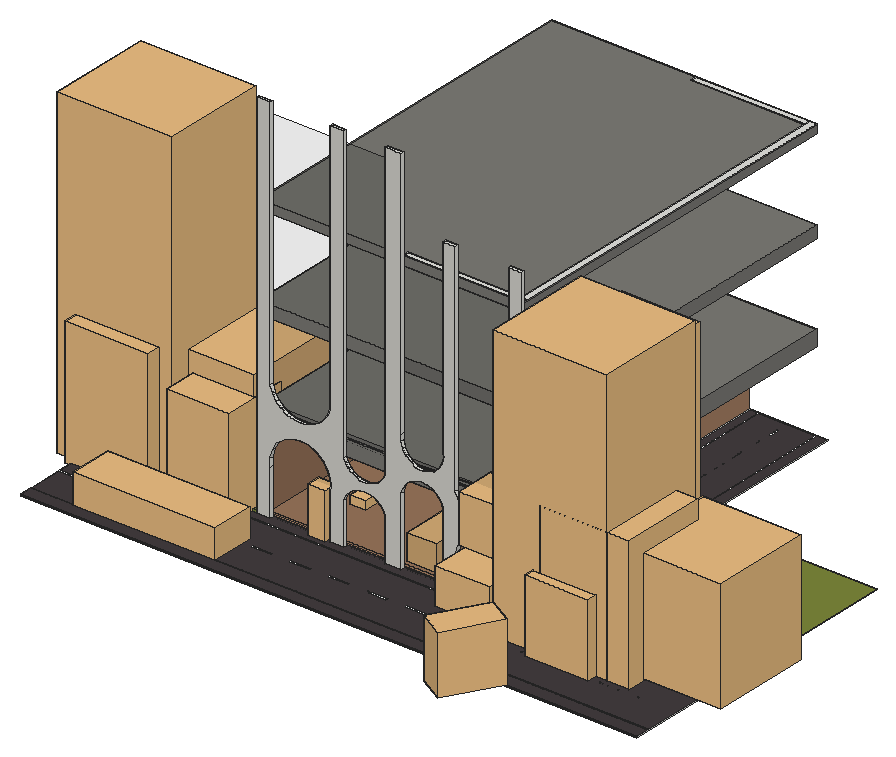
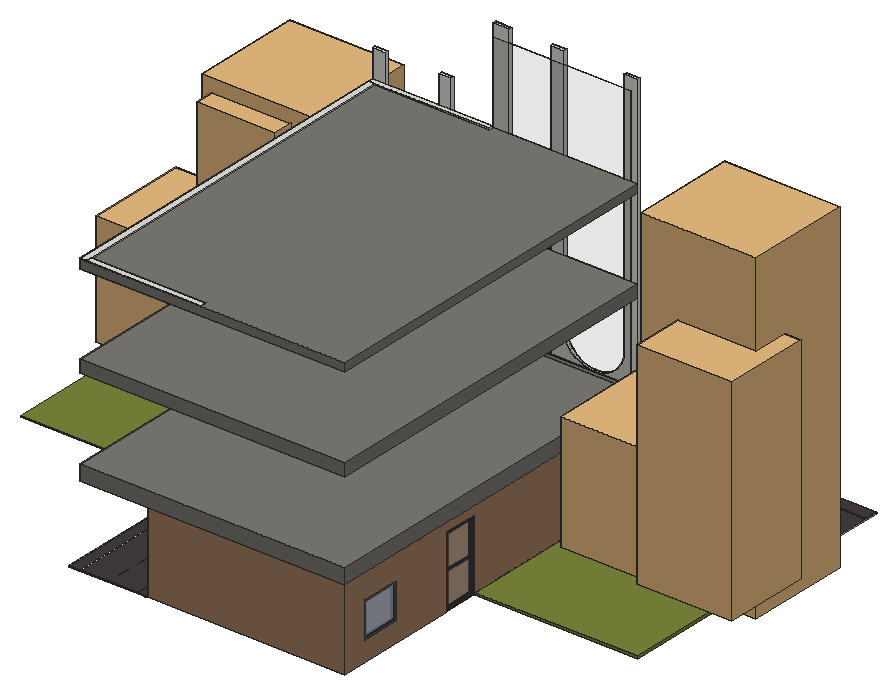
# SketchUp Ruby script. Lengths in inches.
U = 1.inch
M = Sketchup.active_model
def pt(a) = Geom::Point3d.new(a.map { |v| v * U })
def face(e, loops, mat)
  f = e.add_face(loops[0].map { |a| pt(a) })
  loops[1..].each { |l| e.add_face(l.map { |a| pt(a) }).erase! }
  f.material = f.back_material = mat if mat
  f
end
# faces: each face lists its corners as indices into pts; further lists are holes
def faces(e, pts, list, mat = nil) = list.each { |f| face(e, (f[0].is_a?(Array) ? f : [f]).map { |l| l.map { |i| pts[i] } }, mat) }
# xy, xz, yz: faces in a plane at the given z, y or x. An outline is a flat list of corners, or four numbers for a rectangle; further outlines are holes
def ring(l) = l.size == 4 ? [[l[0], l[1]], [l[2], l[1]], [l[2], l[3]], [l[0], l[3]]] : l.each_slice(2).to_a
def flat(e, list, mat, &to3) = list.each { |f| face(e, (f[0].is_a?(Array) ? f : [f]).map { |l| ring(l).map { |u, v| to3.(u, v) } }, mat) }
def xy(e, z, list, mat = nil) = flat(e, list, mat) { |x, y| [x, y, z] }
def xz(e, y, list, mat = nil) = flat(e, list, mat) { |x, z| [x, y, z] }
def yz(e, x, list, mat = nil) = flat(e, list, mat) { |y, z| [x, y, z] }
def lines(e, pts, list) = list.each { |a, b| e.add_line(pt(pts[a]), pt(pts[b])) }
# prism: a flat outline (further loops are holes) pulled along v
def prism(e, loops, v, mat = nil)
  f = face(e, loops, mat); d = Geom::Vector3d.new(v.map { |x| x * U })
  f.pushpull(f.normal.samedirection?(d) ? d.length : -d.length)
end
def box(e, o, s, mat = nil) = prism(e, [[o, [o[0] + s[0], o[1], o[2]], [o[0] + s[0], o[1] + s[1], o[2]], [o[0], o[1] + s[1], o[2]]]], [0, 0, s[2]], mat)
def at(x, y, z, deg = 0) = Geom::Transformation.translation(pt([x, y, z])) * Geom::Transformation.rotation(ORIGIN, Z_AXIS, deg.degrees)
def axes(o, x, y, z) = Geom::Transformation.new([*x, 0, *y, 0, *z, 0, *pt(o).to_a, 1])
def part(name) = M.definitions.add(name)
# library, detail: a bought-in or finely detailed component or shape, given as its bounding box
def library(name, o, s) = part(name).tap { |d| box(d.entities, o, s) }
def detail(e, o, s) = box(e.add_group.entities, o, s)
def put(e, d, t, mat = nil) = e.add_instance(d, t).tap { |i| i.material = mat if mat }
def group(e, t, mat = nil) = e.add_group.tap { |g| g.transformation = t; g.material = mat if mat }.entities
root = M.entities
M.materials.add("Bricks A04 100cm").color = [167, 128, 100]
M.materials.add("Concrete Grey 06 100cm").color = [123, 122, 117]
M.materials.add("Concrete Rough Rocks 16-07 100cm\#1").color = [212, 211, 204]
M.materials.add("Glass Clear 001").color = [0, 0, 0]
M.materials["Glass Clear 001"].alpha = 0.1
M.materials.add("Grass E 200cm\#1").color = [123, 134, 58]
M.materials.add("Windows").color = [58, 58, 58]
M.materials.add("[Asphalt_New]").color = [67, 60, 62]
M.materials.add("[Color_000]").color = [255, 255, 255]
M.materials.add("[Color_006]").color = [86, 86, 86]
M.materials.add("[Translucent Glass Gray]1").color = [128, 128, 128]
M.materials["[Translucent Glass Gray]1"].alpha = 0.5
M.materials.add("[Translucent_Glass_Gray]1").color = [167, 187, 214]
M.materials["[Translucent_Glass_Gray]1"].alpha = 0.8
c1 = library("Schefflera arboricola 004",[-66.29,-60.4,-0.79],[131.92,126.97,148.56])
c2 = library("Schefflera arboricola 003",[-47.85,-46.83,-0.79],[92.88,94.95,107.86])
c3 = part("Window+06")
g1 = group(c3.entities,at(-11,5.5,0,-90))
xy(g1,0,[[0,11,5.5,35]],"Windows")
xy(g1,2,[[0,13,5.5,33]],"Windows")
xy(g1,53,[[0,13,5.5,33]],"Windows")
xy(g1,55,[[0,11,5.5,35]],"Windows")
xz(g1,11,[[0,0,5.5,55]],"Windows")
xz(g1,13,[[0,2,5.5,53]],"Windows")
xz(g1,33,[[0,2,5.5,53]],"Windows")
xz(g1,35,[[0,0,5.5,55]],"Windows")
yz(g1,0,[[[11,0,35,55],[13,2,33,53]]],"Windows")
yz(g1,5.5,[[[11,0,35,55],[13,2,33,53]]],"Windows")
g2 = group(g1,at(2.75,2,2))
xy(g2,0,[[0,11,2,31]],"Windows")
xy(g2,1,[[0,12,1,30],[1,12,2,30]],"Windows")
xy(g2,25,[[0,12,1,30],[1,12,2,30]],"Windows")
xy(g2,26,[[0,11,2,31]],"Windows")
xz(g2,11,[[0,0,2,26]],"Windows")
xz(g2,12,[[0,1,1,25],[1,1,2,25]],"Windows")
xz(g2,30,[[0,1,1,25],[1,1,2,25]],"Windows")
xz(g2,31,[[0,0,2,26]],"Windows")
yz(g2,0,[[[11,0,31,26],[12,1,30,25]]],"Windows")
yz(g2,1,[[12,1,30,25]],"[Translucent Glass Gray]1")
yz(g2,2,[[[11,0,31,26],[12,1,30,25]]],"Windows")
g3 = group(g1,at(0.75,2,27))
xy(g3,0,[[0,11,2,31]],"Windows")
xy(g3,1,[[0,12,1,30],[1,12,2,30]],"Windows")
xy(g3,25,[[0,12,1,30],[1,12,2,30]],"Windows")
xy(g3,26,[[0,11,2,31]],"Windows")
xz(g3,11,[[0,0,2,26]],"Windows")
xz(g3,12,[[0,1,1,25],[1,1,2,25]],"Windows")
xz(g3,30,[[0,1,1,25],[1,1,2,25]],"Windows")
xz(g3,31,[[0,0,2,26]],"Windows")
yz(g3,0,[[[11,0,31,26],[12,1,30,25]]],"Windows")
yz(g3,1,[[12,1,30,25]],"[Translucent Glass Gray]1")
yz(g3,2,[[[11,0,31,26],[12,1,30,25]]],"Windows")
c4 = library("Hugh 001 Standing",[-12.24,-10.14,0],[24.44,20.33,67.86])
c5 = library("Jalen Walking 001",[-18.74,-36.02,0],[37.48,72.04,73.58])
c6 = library("Car 034",[-40.54,-85.05,-1.09],[81.08,168.69,53.52])
c7 = part("Untitled (6)")
xy(c7.entities,0,[[-437.53,-1998.08,-389.53,356.87],[[-383.53,-1998.08,-383.53,356.87,-256.03,356.87,-256.03,283.28,-250.03,283.28,-250.03,356.87,-124.03,356.87,-124.03,-1998.08],[-256.03,136.09,-250.03,209.6875],[-256.03,-158.28,-250.03,-84.68],[-256.03,-599.83,-250.03,-526.24],[-256.03,-11.09,-250.03,62.5],[-256.03,-452.64,-250.03,-379.05],[-256.03,-747.01,-250.03,-673.42],[-256.03,-305.46,-250.03,-231.87],[-256.03,-1630.12,-250.03,-1556.53],[-256.03,-1482.93,-250.03,-1409.34],[-256.03,-1335.75,-250.03,-1262.16],[-256.03,-894.2,-250.03,-820.6],[-256.03,-1924.49,-250.03,-1850.89],[-256.03,-1188.57,-250.03,-1114.97],[-256.03,-1777.3,-250.03,-1703.71],[-256.03,-1041.38,-250.03,-967.79]],[-118.03,-1998.08,-70.03,356.87]],"[Asphalt_New]")
xy(c7.entities,0,[[-389.53,-1998.08,-383.53,356.87],[-124.03,-1998.08,-118.03,356.87],[-256.03,-1924.49,-250.03,-1850.89],[-256.03,-1777.3,-250.03,-1703.71],[-256.03,-1630.12,-250.03,-1556.53],
  [-256.03,-1482.93,-250.03,-1409.34],[-256.03,-1335.75,-250.03,-1262.16],[-256.03,-1188.57,-250.03,-1114.97],[-256.03,-1041.38,-250.03,-967.79],[-256.03,-894.2,-250.03,-820.6],
  [-256.03,-747.01,-250.03,-673.42],[-256.03,-599.83,-250.03,-526.24],[-256.03,-452.64,-250.03,-379.05],[-256.03,-305.46,-250.03,-231.87],[-256.03,-158.28,-250.03,-84.68],
  [-256.03,-11.09,-250.03,62.5],[-256.03,136.09,-250.03,209.6875],[-256.03,283.28,-250.03,356.87]],"[Color_000]")
c8 = library("Reception desk",[23.57,0,0],[37.45,80.71,54.72])
c9 = part("BIC_Bike Shop - Window - Small")
xy(c9.entities,-8,[[[0,0,36,36],[2,2,34,34]]],"[Color_006]")
xy(c9.entities,-4,[[2,2,34,34]],"[Translucent_Glass_Gray]1")
xy(c9.entities,0,[[[0,0,36,36],[2,2,34,34]]],"[Color_006]")
xz(c9.entities,0,[[0,-8,36,0]],"[Color_006]")
xz(c9.entities,2,[[2,-8,34,-4],[2,-4,34,0]],"[Color_006]")
xz(c9.entities,34,[[2,-8,34,-4],[2,-4,34,0]],"[Color_006]")
xz(c9.entities,36,[[0,-8,36,0]],"[Color_006]")
yz(c9.entities,0,[[0,-8,36,0]],"[Color_006]")
yz(c9.entities,2,[[2,-8,34,-4],[2,-4,34,0]],"[Color_006]")
yz(c9.entities,34,[[2,-8,34,-4],[2,-4,34,0]],"[Color_006]")
yz(c9.entities,36,[[0,-8,36,0]],"[Color_006]")
c10 = library("Dome Light",[-12,-12,0],[24,24,12])
c11 = library("Untitled+(35)",[-36.2,-34.81,25.37],[51.5,58.42,71.3])
box(root,[0.025,0,0],[911.788,140.625,1.3125])
box(root,[0,136.481,1.369],[240.0625,305,3.687],"Grass E 200cm\#1")
xy(root,1.369,[[533.3125,141.106,648.125,681.606],[648.125,141.106,648.4375,441.575]])
xy(root,1.369,[[648.4375,141.106,911.8125,441.575]],"Grass E 200cm\#1")
xy(root,2.306,[[533.3125,141.106,648.125,681.606]])
xy(root,3.056,[[648.4375,141.106,911.8125,441.575]],"Grass E 200cm\#1")
xy(root,140.053,[[247.445,141.106,612.5,150.106]],"Glass Clear 001")
xy(root,144.302,[[249.0625,141.606,453.445,141.606,612.5,150.106,247.445,150.106]],"Glass Clear 001")
xy(root,414.5625,[[631.5625,141.106,622.077,148.731,631.5625,148.731]])
xy(root,416.25,[[453.5,141.106,631.5625,141.106,631.5625,148.732,622.077,148.732,453.5,148.731]])
xy(root,534.5625,[[249.0625,141.106,453.445,141.606]],"Glass Clear 001")
xz(root,140.883,[[453.5,141.727,612.5,401.8125]],"Glass Clear 001")
xz(root,141.106,[[533.3125,1.369,648.125,2.306]])
xz(root,141.106,[[631.5625,414.5625,631.5625,416.25,453.5,416.25]],"Concrete Grey 06 100cm")
xz(root,141.106,[[247.445,140.053,249.0625,140.053,247.445,144.302]],"Glass Clear 001")
xz(root,141.606,[[249.0625,144.302,453.445,534.5625]],"Glass Clear 001")
xz(root,144.219,[[248.63,1.8125,513.626,119.9375]],"Glass Clear 001")
xz(root,148.731,[[622.077,414.5625,631.5625,414.929]])
xz(root,148.732,[[622.077,415.0625,631.5625,416.25]])
xz(root,150.106,[[247.445,140.053,612.5,144.302]],"Glass Clear 001")
xz(root,441.575,[[648.4375,1.369,911.8125,3.056]],"Grass E 200cm\#1")
xz(root,681.606,[[533.3125,1.369,648.125,2.306]])
yz(root,247.445,[[141.106,140.053,150.106,144.302]],"Glass Clear 001")
yz(root,249.0625,[[141.106,140.053,141.106,534.5625,141.606,534.5625,141.606,144.302]],"Glass Clear 001")
yz(root,453.445,[[141.106,140.053,141.606,144.302,141.606,534.5625,141.106,534.5625]],"Glass Clear 001")
yz(root,453.5,[[140.883,401.8125,141.106,416.25,148.731,416.25,148.731,414.5625]])
yz(root,533.3125,[[141.106,1.369,681.606,2.306]])
yz(root,612.5,[[141.106,140.053,150.106,140.053,150.106,144.302,140.883,141.727]],"Glass Clear 001")
yz(root,622.077,[[681.105,413.821,148.731,414.5625,148.731,414.929,148.732,415.0625,148.733,416.25,672.071,415.521,680.233,415.51,681.107,415.509,681.106,414.635]])
yz(root,631.5625,[[681.105,413.821,681.107,415.509,148.733,416.25,148.732,415.0625,148.731,414.929,148.731,414.5625],[141.106,414.5625,148.731,414.5625,148.731,414.929,148.732,415.0625,148.732,416.25,141.106,416.25]],"Concrete Grey 06 100cm")
yz(root,648.125,[[141.106,1.369,681.606,2.306]])
yz(root,648.4375,[[141.106,1.369,441.575,3.056]],"Grass E 200cm\#1")
p = [[453.445,141.106,140.053],[453.5,140.883,141.727],[453.445,141.606,144.302],[453.5,141.106,140.053],[612.5,141.106,140.053],[612.5,140.883,141.727],
  [247.445,141.106,144.302],[249.0625,141.106,140.053],[247.445,150.106,144.302],[249.0625,141.606,144.302],[612.5,150.106,144.302],[453.5,140.883,401.8125],
  [453.5,148.731,414.5625],[622.077,148.731,414.5625],[612.5,140.883,401.8125],[622.082,672.069,414.648],[453.817,672.068,413.701],[453.817,681.105,413.689],
  [622.077,681.106,414.635],[622.082,681.106,414.635],[622.082,680.232,414.636],[622.077,672.071,415.521],[453.8125,672.069,414.575],[453.8125,681.106,414.5625],
  [622.077,681.107,415.509],[622.077,681.105,413.821],[631.5625,681.105,413.821],[631.5625,148.731,414.5625],[631.5625,681.107,415.509],[622.077,148.731,414.929],
  [631.5625,148.731,414.929],[453.5,148.731,416.25],[622.077,148.732,416.25],[622.077,148.732,415.0625],[622.077,680.233,415.51],[631.5625,148.732,415.0625],
  [631.5625,148.733,416.25],[622.077,148.733,416.25],[0,-122.738,5.056],[0,-122.738,1.744]]
faces(root,p,[[0,1,2],[1,0,3],[3,4,5,1],[6,7,8],[9,8,7],[0,2,9,7],[1,10,2],[5,10,1]],"Glass Clear 001")
faces(root,p,[[11,12,13,14],[15,16,17,18,19,20],[21,22,16,15],[22,23,17,16],[23,24,18,17],[13,25,26,27],[25,18,19,24,28,26],[29,30,27,13,12,31,32,33],
  [22,21,34,24,23],[34,21,15,20],[24,34,20,19],[18,24,19],[29,30,35,33],[33,35,36,37],[34,21,37,36,28,24]])
lines(root,p,[[38,39]])
put(root,c1,axes([688.01,171.53,-13.56],[0.7936,0,0],[0,0.7936,0],[0,0,1.69965]))
put(root,c1,axes([47.65,188.84,-5.3],[1.2932,0,0],[0,1.22,0],[0,0,3.2208]))
put(root,c1,axes([769.6,141.11,0.27],[1,0,0],[0,1,0],[0,0,1.34]))
put(root,c1,axes([151.57,215.65,0.16],[1.2,0,0],[0,1.2,0],[0,0,1.2]))
put(root,c2,axes([53.78,141.01,0.58],[1.32,0,0],[0,1,0],[0,0,1.73203]))
put(root,c2,axes([188.3,141.01,0.31],[1,0,0],[0,1,0],[0,0,1.39]))
put(root,c1,axes([718.9,158.02,1.8125],[1.28,0,0],[0,1.28,0],[0,0,2.74138]))
put(root,c2,at(740.74,113.62,2))
put(root,c3,axes([242.3125,494.89,1.37],[0,-2.22917,0],[0.375,0,0],[0,0,1.92841]))
g4 = group(root,at(138.3125,141.11,0))
xy(g4,1.37,[[377.5625,-0.5,377.5625,531,110.75,531,110.75,353.78,101.75,353.78,101.75,540,393.52,540,393.52,-0.5],[101.75,0,110.75,300.47],[110.75,0,377.5625,9],[110.75,9,377.5625,531]],"Bricks A04 100cm")
xy(g4,30.4375,[[101.75,444.5,110.75,505.8125]],"Bricks A04 100cm")
xy(g4,85.12,[[101.75,444.5,110.75,505.8125]],"Bricks A04 100cm")
xy(g4,108.18,[[101.75,300.47,110.75,353.78]],"Bricks A04 100cm")
xy(g4,119.99,[[377.5625,-0.5,393.52,-0.5,393.52,540,101.75,540,101.75,0,110.75,0,110.75,531,377.5625,531]],"Bricks A04 100cm")
xz(g4,-0.5,[[377.5625,1.37,393.52,119.99]],"Bricks A04 100cm")
xz(g4,0,[[101.75,1.37,110.75,119.99]],"Bricks A04 100cm")
xz(g4,300.47,[[101.75,1.37,110.75,108.18]],"Bricks A04 100cm")
xz(g4,353.78,[[101.75,1.37,110.75,108.18]],"Bricks A04 100cm")
xz(g4,444.5,[[101.75,30.4375,110.75,85.12]],"Bricks A04 100cm")
xz(g4,505.8125,[[101.75,30.4375,110.75,85.12]],"Bricks A04 100cm")
xz(g4,531,[[110.75,1.37,377.5625,119.99]],"Bricks A04 100cm")
xz(g4,540,[[101.75,1.37,393.52,119.99]],"Bricks A04 100cm")
yz(g4,101.75,[[[0,1.37,0,119.99,540,119.99,540,1.37,353.78,1.37,353.78,108.18,300.47,108.18,300.47,1.37],[444.5,30.4375,505.8125,85.12]]],"Bricks A04 100cm")
yz(g4,110.75,[[0,1.37,9,119.99],[[9,1.37,300.47,1.37,300.47,108.18,353.78,108.18,353.78,1.37,531,1.37,531,119.99,9,119.99],[444.5,30.4375,505.8125,85.12]]],"Bricks A04 100cm")
yz(g4,377.5625,[[-0.5,1.37,531,119.99]],"Bricks A04 100cm")
yz(g4,393.52,[[-0.5,1.37,540,119.99]],"Bricks A04 100cm")
g5 = group(root,at(1099.8125,-728.61,1.37))
xy(g5,0,[[-859.75,865.09,-839.625,869.72],[-750.875,865.09,-731,869.72],[-669.5625,865.09,-646,869.72],[-584.125,865.09,-566.5,869.72]])
xy(g5,455.76,[[-584.125,865.09,-566.1875,869.72],[-487.75,865.09,-468,869.72]])
xy(g5,550.82,[[-859.75,865.09,-839.625,869.72],[-750.875,865.09,-731,869.72],[-669.5625,865.09,-646,869.72]])
xz(g5,865.09,[[-859.75,0,-839.625,0,-839.625,66.75,-839.78,79.63,-836.27,92.02,-829.38,102.91,-819.69,111.4,-808,116.78,-795.25,118.63,-782.5,116.78,-770.8,111.4,-761.11,102.91,-754.23,92.02,-750.72,79.63,-750.875,66.75,-750.875,0,-731,0,-731,62.4375,-728.15,68.47,-724.125,73.8,-719.1,78.2,-713.28,81.48,-706.92,83.5,-700.28,84.1875,-693.64,83.5,-687.28,81.48,-681.46,78.2,-676.4375,73.8,-672.41,68.47,-669.5625,62.4375,-669.5625,0,-646,0,-646,101.625,-643.7,108.39,-639.95,114.47,-634.93,119.55,-628.9,123.38,-622.16,125.76,-615.0625,126.5625,-607.96,125.76,-601.23,123.38,-595.19,119.55,-590.17,114.47,-586.42,108.39,-584.125,101.625,-584.125,0,-566.5,0,-566.5,38.9375,-565.37,50.2,-562.02,61.02,-556.6,70.95,-549.31,79.61,-540.44,86.65,-530.36,91.79,-519.45,94.82,-508.16,95.625,-496.94,94.17,-486.22,90.52,-476.45,84.8125,-468,77.28,-468,455.76,-487.75,455.76,-487.75,132.21,-491.16,124.22,-496.1875,117.13,-502.59,111.26,-510.08,106.87,-518.33,104.15,-526.97,103.23,-535.61,104.15,-543.86,106.87,-551.35,111.26,-557.75,117.13,-562.77,124.22,-566.1875,132.21,-566.1875,455.76,-584.125,455.76,-584.125,179.13,-583.7,169.91,-585.97,160.96,-590.73,153.05,-597.58,146.86,-605.93,142.92,-615.0625,141.57,-624.19,142.92,-632.54,146.86,-639.39,153.05,-644.16,160.96,-646.42,169.91,-646,179.13,-646,550.82,-669.5625,550.82,-669.5625,118.63,-672.23,112.36,-676.15,106.8,-681.17,102.1875,-687.04,98.74,-693.51,96.6,-700.28,95.88,-707.05,96.6,-713.52,98.74,-719.39,102.1875,-724.41,106.8,-728.33,112.36,-731,118.63,-731,550.82,-750.875,550.82,-750.875,176.63,-754.3,167.08,-759.76,158.53,-766.97,151.39,-775.58,146.03,-785.17,142.7,-795.25,141.57,-805.33,142.7,-814.92,146.03,-823.53,151.39,-830.74,158.53,-836.19,167.08,-839.625,176.63,-839.625,550.82,-859.75,550.82]],"Concrete Rough Rocks 16-07 100cm\#1")
xz(g5,869.72,[[-859.75,0,-859.75,550.82,-839.625,550.82,-839.625,176.63,-836.19,167.08,-830.74,158.53,-823.53,151.39,-814.92,146.03,-805.33,142.7,-795.25,141.57,-785.17,142.7,-775.58,146.03,-766.97,151.39,-759.76,158.53,-754.3,167.08,-750.875,176.63,-750.875,550.82,-731,550.82,-731,118.63,-728.33,112.36,-724.41,106.8,-719.39,102.1875,-713.52,98.74,-707.05,96.6,-700.28,95.88,-693.51,96.6,-687.04,98.74,-681.17,102.1875,-676.15,106.8,-672.23,112.36,-669.5625,118.63,-669.5625,550.82,-646,550.82,-646,179.13,-646.42,169.91,-644.16,160.96,-639.39,153.05,-632.54,146.86,-624.19,142.92,-615.0625,141.57,-605.93,142.92,-597.58,146.86,-590.73,153.05,-585.97,160.96,-583.7,169.91,-584.125,179.13,-584.125,455.76,-566.1875,455.76,-566.1875,132.21,-562.77,124.22,-557.75,117.13,-551.35,111.26,-543.86,106.87,-535.61,104.15,-526.97,103.23,-518.33,104.15,-510.08,106.87,-502.59,111.26,-496.1875,117.13,-491.16,124.22,-487.75,132.21,-487.75,455.76,-468,455.76,-468,77.28,-476.45,84.8125,-486.22,90.52,-496.94,94.17,-508.16,95.625,-519.45,94.82,-530.36,91.79,-540.44,86.65,-549.31,79.61,-556.6,70.95,-562.02,61.02,-565.37,50.2,-566.5,38.9375,-566.5,0,-584.125,0,-584.125,101.625,-586.42,108.39,-590.17,114.47,-595.19,119.55,-601.23,123.38,-607.96,125.76,-615.0625,126.5625,-622.16,125.76,-628.9,123.38,-634.93,119.55,-639.95,114.47,-643.7,108.39,-646,101.625,-646,0,-669.5625,0,-669.5625,62.4375,-672.41,68.47,-676.4375,73.8,-681.46,78.2,-687.28,81.48,-693.64,83.5,-700.28,84.1875,-706.92,83.5,-713.28,81.48,-719.1,78.2,-724.125,73.8,-728.15,68.47,-731,62.4375,-731,0,-750.875,0,-750.875,66.75,-750.72,79.63,-754.23,92.02,-761.11,102.91,-770.8,111.4,-782.5,116.78,-795.25,118.63,-808,116.78,-819.69,111.4,-829.38,102.91,-836.27,92.02,-839.78,79.63,-839.625,66.75,-839.625,0]])
yz(g5,-859.75,[[865.09,0,869.72,550.82]])
yz(g5,-839.625,[[865.09,0,869.72,66.75],[865.09,176.63,869.72,550.82]])
yz(g5,-750.875,[[865.09,0,869.72,66.75],[865.09,176.63,869.72,550.82]])
yz(g5,-731,[[865.09,0,869.72,62.4375],[865.09,118.63,869.72,550.82]])
yz(g5,-669.5625,[[865.09,0,869.72,62.4375],[865.09,118.63,869.72,550.82]])
yz(g5,-646,[[865.09,0,869.72,101.625],[865.09,179.13,869.72,550.82]])
yz(g5,-584.125,[[865.09,0,869.72,101.625],[865.09,179.13,869.72,455.76]])
yz(g5,-566.5,[[865.09,0,869.72,38.9375]])
yz(g5,-566.1875,[[865.09,132.21,869.72,455.76]])
yz(g5,-487.75,[[865.09,132.21,869.72,455.76]])
yz(g5,-468,[[865.09,77.28,869.72,455.76]])
p = [[-565.37,865.09,50.2],[-566.5,865.09,38.9375],[-566.5,869.72,38.9375],[-565.37,869.72,50.2],[-562.02,865.09,61.02],[-562.02,869.72,61.02],
  [-556.6,865.09,70.95],[-556.6,869.72,70.95],[-728.15,869.72,68.47],[-728.15,865.09,68.47],[-731,865.09,62.4375],[-731,869.72,62.4375],
  [-669.5625,869.72,62.4375],[-669.5625,865.09,62.4375],[-672.41,865.09,68.47],[-672.41,869.72,68.47],[-839.78,869.72,79.63],[-839.78,865.09,79.63],
  [-839.625,865.09,66.75],[-839.625,869.72,66.75],[-750.875,869.72,66.75],[-750.875,865.09,66.75],[-750.72,865.09,79.63],[-750.72,869.72,79.63],
  [-724.125,869.72,73.8],[-724.125,865.09,73.8],[-676.4375,865.09,73.8],[-676.4375,869.72,73.8],[-549.31,865.09,79.61],[-549.31,869.72,79.61],
  [-719.1,869.72,78.2],[-719.1,865.09,78.2],[-681.46,865.09,78.2],[-681.46,869.72,78.2],[-468,865.09,77.28],[-476.45,865.09,84.8125],
  [-476.45,869.72,84.8125],[-468,869.72,77.28],[-713.28,869.72,81.48],[-713.28,865.09,81.48],[-687.28,865.09,81.48],[-687.28,869.72,81.48],
  [-836.27,869.72,92.02],[-836.27,865.09,92.02],[-754.23,865.09,92.02],[-754.23,869.72,92.02],[-540.44,865.09,86.65],[-540.44,869.72,86.65],
  [-706.92,869.72,83.5],[-706.92,865.09,83.5],[-693.64,865.09,83.5],[-693.64,869.72,83.5],[-700.28,869.72,84.1875],[-700.28,865.09,84.1875],
  [-486.22,865.09,90.52],[-486.22,869.72,90.52],[-530.36,865.09,91.79],[-530.36,869.72,91.79],[-496.94,865.09,94.17],[-496.94,869.72,94.17],
  [-519.45,865.09,94.82],[-519.45,869.72,94.82],[-829.38,869.72,102.91],[-829.38,865.09,102.91],[-761.11,865.09,102.91],[-761.11,869.72,102.91],
  [-508.16,865.09,95.625],[-508.16,869.72,95.625],[-707.05,869.72,96.6],[-707.05,865.09,96.6],[-700.28,865.09,95.88],[-700.28,869.72,95.88],
  [-693.51,865.09,96.6],[-693.51,869.72,96.6],[-713.52,869.72,98.74],[-713.52,865.09,98.74],[-687.04,865.09,98.74],[-687.04,869.72,98.74],
  [-719.39,869.72,102.1875],[-719.39,865.09,102.1875],[-681.17,865.09,102.1875],[-681.17,869.72,102.1875],[-643.7,869.72,108.39],[-643.7,865.09,108.39],
  [-646,865.09,101.625],[-646,869.72,101.625],[-584.125,869.72,101.625],[-584.125,865.09,101.625],[-586.42,865.09,108.39],[-586.42,869.72,108.39],
  [-724.41,869.72,106.8],[-724.41,865.09,106.8],[-676.15,865.09,106.8],[-676.15,869.72,106.8],[-819.69,869.72,111.4],[-819.69,865.09,111.4],
  [-770.8,865.09,111.4],[-770.8,869.72,111.4],[-535.61,869.72,104.15],[-535.61,865.09,104.15],[-526.97,865.09,103.23],[-526.97,869.72,103.23],
  [-518.33,865.09,104.15],[-518.33,869.72,104.15],[-543.86,869.72,106.87],[-543.86,865.09,106.87],[-510.08,865.09,106.87],[-510.08,869.72,106.87],
  [-728.33,869.72,112.36],[-728.33,865.09,112.36],[-672.23,865.09,112.36],[-672.23,869.72,112.36],[-551.35,869.72,111.26],[-551.35,865.09,111.26],
  [-502.59,865.09,111.26],[-502.59,869.72,111.26],[-639.95,869.72,114.47],[-639.95,865.09,114.47],[-590.17,865.09,114.47],[-590.17,869.72,114.47],
  [-557.75,869.72,117.13],[-557.75,865.09,117.13],[-496.1875,865.09,117.13],[-496.1875,869.72,117.13],[-808,869.72,116.78],[-808,865.09,116.78],
  [-782.5,865.09,116.78],[-782.5,869.72,116.78],[-731,869.72,118.63],[-731,865.09,118.63],[-669.5625,865.09,118.63],[-669.5625,869.72,118.63],
  [-634.93,869.72,119.55],[-634.93,865.09,119.55],[-595.19,865.09,119.55],[-595.19,869.72,119.55],[-795.25,869.72,118.63],[-795.25,865.09,118.63],
  [-562.77,869.72,124.22],[-562.77,865.09,124.22],[-491.16,865.09,124.22],[-491.16,869.72,124.22],[-628.9,869.72,123.38],[-628.9,865.09,123.38],
  [-601.23,865.09,123.38],[-601.23,869.72,123.38],[-622.16,869.72,125.76],[-622.16,865.09,125.76],[-607.96,865.09,125.76],[-607.96,869.72,125.76],
  [-566.1875,869.72,132.21],[-566.1875,865.09,132.21],[-487.75,865.09,132.21],[-487.75,869.72,132.21],[-615.0625,869.72,126.5625],[-615.0625,865.09,126.5625],
  [-805.33,869.72,142.7],[-805.33,865.09,142.7],[-795.25,865.09,141.57],[-795.25,869.72,141.57],[-785.17,865.09,142.7],[-785.17,869.72,142.7],
  [-624.19,869.72,142.92],[-624.19,865.09,142.92],[-615.0625,865.09,141.57],[-615.0625,869.72,141.57],[-605.93,865.09,142.92],[-605.93,869.72,142.92],
  [-814.92,869.72,146.03],[-814.92,865.09,146.03],[-775.58,865.09,146.03],[-775.58,869.72,146.03],[-632.54,869.72,146.86],[-632.54,865.09,146.86],
  [-597.58,865.09,146.86],[-597.58,869.72,146.86],[-823.53,869.72,151.39],[-823.53,865.09,151.39],[-766.97,865.09,151.39],[-766.97,869.72,151.39],
  [-639.39,869.72,153.05],[-639.39,865.09,153.05],[-590.73,865.09,153.05],[-590.73,869.72,153.05],[-830.74,869.72,158.53],[-830.74,865.09,158.53],
  [-759.76,865.09,158.53],[-759.76,869.72,158.53],[-644.16,869.72,160.96],[-644.16,865.09,160.96],[-585.97,865.09,160.96],[-585.97,869.72,160.96],
  [-836.19,869.72,167.08],[-836.19,865.09,167.08],[-754.3,865.09,167.08],[-754.3,869.72,167.08],[-646.42,869.72,169.91],[-646.42,865.09,169.91],
  [-583.7,865.09,169.91],[-583.7,869.72,169.91],[-839.625,869.72,176.63],[-839.625,865.09,176.63],[-750.875,865.09,176.63],[-750.875,869.72,176.63],
  [-646,869.72,179.13],[-646,865.09,179.13],[-584.125,865.09,179.13],[-584.125,869.72,179.13],[-584.125,872.65,179.13]]
faces(g5,p,[[0,1,2,3],[4,0,3,5],[6,4,5,7],[8,9,10,11],[12,13,14,15],[16,17,18,19],[20,21,22,23],[24,25,9,8],
  [15,14,26,27],[28,6,7,29],[30,31,25,24],[27,26,32,33],[34,35,36,37],[38,39,31,30],[33,32,40,41],[42,43,17,16],
  [23,22,44,45],[46,28,29,47],[48,49,39,38],[41,40,50,51],[52,53,49,48],[51,50,53,52],[35,54,55,36],[56,46,47,57],
  [54,58,59,55],[60,56,57,61],[62,63,43,42],[45,44,64,65],[58,66,67,59],[66,60,61,67],[68,69,70,71],[71,70,72,73],
  [74,75,69,68],[73,72,76,77],[78,79,75,74],[77,76,80,81],[82,83,84,85],[86,87,88,89],[90,91,79,78],[81,80,92,93],
  [94,95,63,62],[65,64,96,97],[98,99,100,101],[101,100,102,103],[104,105,99,98],[103,102,106,107],[108,109,91,90],[93,92,110,111],
  [112,113,105,104],[107,106,114,115],[116,117,83,82],[89,88,118,119],[120,121,113,112],[115,114,122,123],[124,125,95,94],[97,96,126,127],
  [128,129,109,108],[111,110,130,131],[132,133,117,116],[119,118,134,135],[136,137,125,124],[127,126,137,136],[138,139,121,120],[123,122,140,141],
  [142,143,133,132],[135,134,144,145],[146,147,143,142],[145,144,148,149],[150,151,139,138],[141,140,152,153],[154,155,147,146],[149,148,155,154],
  [156,157,158,159],[159,158,160,161],[162,163,164,165],[165,164,166,167],[168,169,157,156],[161,160,170,171],[172,173,163,162],[167,166,174,175],
  [176,177,169,168],[171,170,178,179],[180,181,173,172],[175,174,182,183],[184,185,177,176],[179,178,186,187],[188,189,181,180],[183,182,190,191],
  [192,193,185,184],[187,186,194,195],[196,197,189,188],[191,190,198,199],[200,201,193,192],[195,194,202,203],[204,205,197,196],[199,198,206,207]])
lines(g5,p,[[207,208]])
put(root,c4,at(331.68,142.22,1.8125))
put(root,c5,axes([678.13,-25.75,1.8125],[1.02191,-0.59,0],[0.59,1.02191,0],[0,0,1.18]))
put(root,c6,axes([166.68,51.01,2.6875],[0,0.8,0],[-1.24544,0,0],[0,0,0.8]))
put(root,c6,axes([578.39,225.59,2.9],[1,0,0],[0,1.5568,0],[0,0,1]))
put(root,c7,axes([138.56,169.33,1.8125],[0,0.387,0],[-0.387,0,0],[0,0,0.387]))
put(root,c7,axes([508.3,222.75,2.31],[-0.31958,0,0],[0,-0.22878,0],[0,0,0.279]))
put(root,c2,axes([880.67,178.68,6.27],[1.5525,0,0],[0,1.5525,0],[0,0,1.53883]))
put(root,c2,axes([829.43,174.43,11],[1.15,0,0],[0,1.15,0],[0,0,1.15]))
put(root,c8,axes([427.63,144.22,10.13],[1.18,0,0],[0,1.18,0],[0,0,0.6844]))
put(root,c8,axes([427.63,267.59,10.13],[1.18,0,0],[0,1.18,0],[0,0,0.6844]))
put(root,c1,axes([729.37,205.53,13.51],[0.88,0,0],[0,1,0],[0,0,2.5311]))
put(root,c9,axes([240.0625,646.92,30.4375],[0,-1.70312,0],[0,0,1.50107],[-0.5763,0,0]))
put(root,c1,axes([7.82,278.72,32.9375],[1.06,0,0],[0,1,0],[0,0,2.1296]))
put(root,c10,at(399.53,136.48,70.56))
put(root,c11,at(594.36,146.97,55.58))
g6 = group(root,at(-660.5625,139.09,143))
box(g6,[900.625,2.02,119.9375],[391.5,540,18.875],"Concrete Grey 06 100cm")
box(g6,[900.625,2.02,258.8125],[391.5,540,12.75],"Concrete Grey 06 100cm")
xy(g6,-39.4375,[[1193.07,2.02,1275.63,5.83]],"Concrete Grey 06 100cm")
xy(g6,-23.0625,[[900.625,2.02,900.625,542.02,1292.125,542.02,1292.125,2.02,1275.63,2.02,1275.63,5.83,1193.07,5.83,1193.07,2.02]],"Concrete Grey 06 100cm")
xy(g6,-0.0625,[[900.625,2.02,1292.125,542.02]],"Concrete Grey 06 100cm")
xz(g6,2.02,[[1193.07,-39.4375,1275.63,-39.4375,1275.63,-23.0625,1292.125,-23.0625,1292.125,-0.0625,900.625,-0.0625,900.625,-23.0625,1193.07,-23.0625]],"Concrete Grey 06 100cm")
xz(g6,5.83,[[1193.07,-39.4375,1275.63,-23.0625]],"Concrete Grey 06 100cm")
xz(g6,542.02,[[900.625,-23.0625,1292.125,-0.0625]],"Concrete Grey 06 100cm")
yz(g6,900.625,[[2.02,-23.0625,542.02,-0.0625]],"Concrete Grey 06 100cm")
yz(g6,1193.07,[[2.02,-39.4375,5.83,-23.0625]],"Concrete Grey 06 100cm")
yz(g6,1275.63,[[2.02,-39.4375,5.83,-23.0625]],"Concrete Grey 06 100cm")
yz(g6,1292.125,[[2.02,-23.0625,542.02,-0.0625]],"Concrete Grey 06 100cm")
